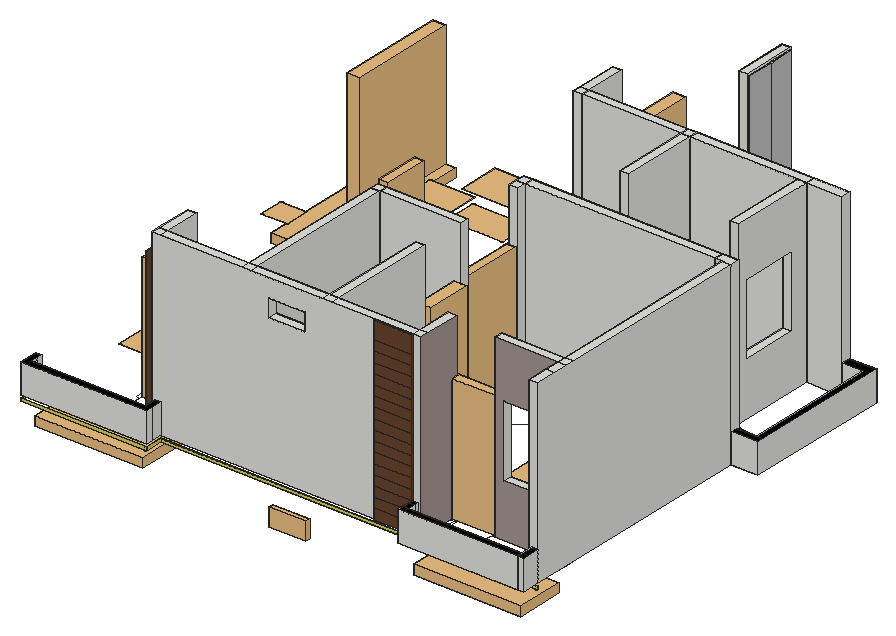
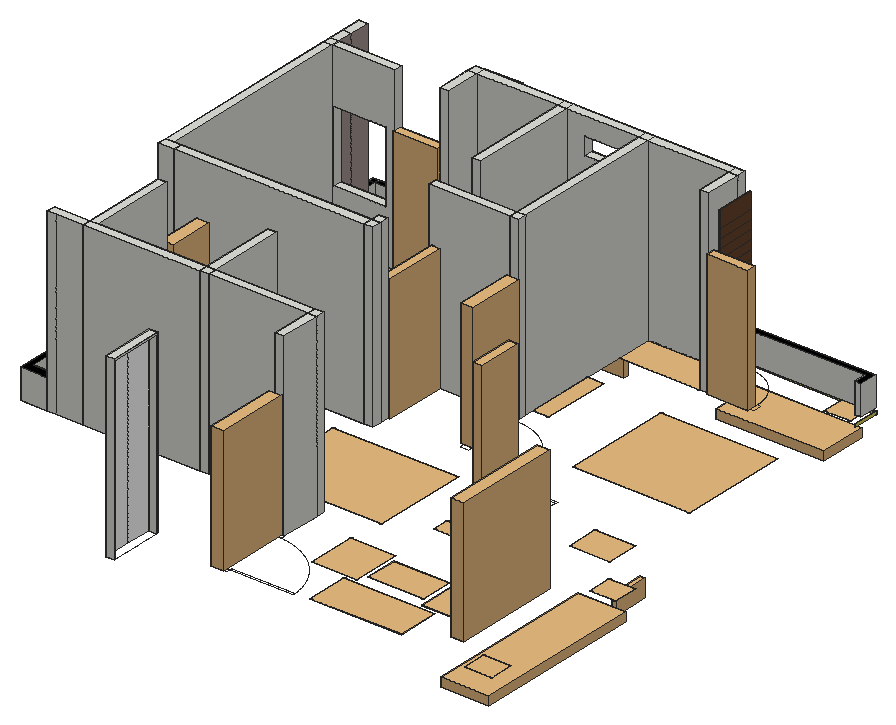
# SketchUp Ruby script. Lengths in inches.
U = 1.inch
M = Sketchup.active_model
def pt(a) = Geom::Point3d.new(a.map { |v| v * U })
def face(e, loops, mat)
  f = e.add_face(loops[0].map { |a| pt(a) })
  loops[1..].each { |l| e.add_face(l.map { |a| pt(a) }).erase! }
  f.material = f.back_material = mat if mat
  f
end
# faces: each face lists its corners as indices into pts; further lists are holes
def faces(e, pts, list, mat = nil) = list.each { |f| face(e, (f[0].is_a?(Array) ? f : [f]).map { |l| l.map { |i| pts[i] } }, mat) }
# xy, xz, yz: faces in a plane at the given z, y or x. An outline is a flat list of corners, or four numbers for a rectangle; further outlines are holes
def ring(l) = l.size == 4 ? [[l[0], l[1]], [l[2], l[1]], [l[2], l[3]], [l[0], l[3]]] : l.each_slice(2).to_a
def flat(e, list, mat, &to3) = list.each { |f| face(e, (f[0].is_a?(Array) ? f : [f]).map { |l| ring(l).map { |u, v| to3.(u, v) } }, mat) }
def xy(e, z, list, mat = nil) = flat(e, list, mat) { |x, y| [x, y, z] }
def xz(e, y, list, mat = nil) = flat(e, list, mat) { |x, z| [x, y, z] }
def yz(e, x, list, mat = nil) = flat(e, list, mat) { |y, z| [x, y, z] }
def lines(e, pts, list) = list.each { |a, b| e.add_line(pt(pts[a]), pt(pts[b])) }
# prism: a flat outline (further loops are holes) pulled along v
def prism(e, loops, v, mat = nil)
  f = face(e, loops, mat); d = Geom::Vector3d.new(v.map { |x| x * U })
  f.pushpull(f.normal.samedirection?(d) ? d.length : -d.length)
end
def box(e, o, s, mat = nil) = prism(e, [[o, [o[0] + s[0], o[1], o[2]], [o[0] + s[0], o[1] + s[1], o[2]], [o[0], o[1] + s[1], o[2]]]], [0, 0, s[2]], mat)
def at(x, y, z, deg = 0) = Geom::Transformation.translation(pt([x, y, z])) * Geom::Transformation.rotation(ORIGIN, Z_AXIS, deg.degrees)
def axes(o, x, y, z) = Geom::Transformation.new([*x, 0, *y, 0, *z, 0, *pt(o).to_a, 1])
def part(name) = M.definitions.add(name)
# library, detail: a bought-in or finely detailed component or shape, given as its bounding box
def library(name, o, s) = part(name).tap { |d| box(d.entities, o, s) }
def detail(e, o, s) = box(e.add_group.entities, o, s)
def put(e, d, t, mat = nil) = e.add_instance(d, t).tap { |i| i.material = mat if mat }
def group(e, t, mat = nil) = e.add_group.tap { |g| g.transformation = t; g.material = mat if mat }.entities
root = M.entities
M.materials.add("0-SS4").color = [255, 255, 255]
M.materials.add("0-SS7").color = [192, 192, 192]
M.materials.add("0-grey 3").color = [204, 204, 204]
M.materials.add("2121 AP  X165 Dhaani-I").color = [217, 210, 92]
M.materials.add("M09_Shadow_Night").color = [0, 0, 0]
M.materials.add("Marble_06_1K").color = [165, 150, 147]
M.materials.add("Wood_Veneer_15_1K").color = [103, 69, 45]
c1 = part("Group\#6")
xy(c1.entities,0,[[0,-8,80,-4],[80,-8,84,-4],[0,-4,4,0],[80,-4,84,4],[0,0,4,4]])
xy(c1.entities,20,[[0,-8,84,-8,84,4,80,4,80,-4,4,-4,4,4,0,4]],"M09_Shadow_Night")
xz(c1.entities,-8,[[0,0,84,20]])
xz(c1.entities,-4,[[4,0,80,20]])
xz(c1.entities,4,[[0,0,4,20],[80,0,84,20]])
yz(c1.entities,0,[[-8,0,4,20]])
yz(c1.entities,4,[[-4,0,0,20],[0,0,4,20]])
yz(c1.entities,80,[[-4,0,4,20]])
yz(c1.entities,84,[[-8,0,-4,20],[-4,0,4,20]])
c2 = part("Group\#8")
xy(c2.entities,0,[[0,-8.88,4,-4.88],[4,-8.88,80,-4.88],[80,-8.88,84,-4.88],[0,-4.88,4,0],[80,-4.88,84,3.12],
  [0,0,4,3.12]])
xy(c2.entities,20,[[0,-8.88,4,-4.88],[4,-8.88,80,-4.88],[80,-8.88,84,-4.88],[0,-4.88,4,0],[80,-4.88,84,3.12],
  [0,0,4,3.12]],"M09_Shadow_Night")
xz(c2.entities,-8.88,[[0,0,80,20],[80,0,84,20]])
xz(c2.entities,-4.88,[[4,0,80,20]])
xz(c2.entities,3.12,[[0,0,4,20],[80,0,84,20]])
yz(c2.entities,0,[[-8.88,0,3.12,20]])
yz(c2.entities,4,[[-4.88,0,0,20],[0,0,3.12,20]])
yz(c2.entities,80,[[-8.88,0,-4.88,20],[-4.88,0,3.12,20]])
yz(c2.entities,84,[[-8.88,0,3.12,20]])
c3 = part("Group\#144")
xy(c3.entities,0,[[0,0,84.5,0.1],[84.5,0,84.6,0.1],[0,0.1,0.5,17.21],[84.5,0.1,84.5,12.09,336.84,12.09,336.84,11.99,84.6,11.99,84.6,0.1]])
xy(c3.entities,2,[[0,0,84.5,0.1],[84.5,0,84.6,0.1],[0,0.1,0.5,17.21],[84.5,0.1,84.6,0.1,84.6,11.99,336.84,11.99,336.84,12.09,84.5,12.09]])
xz(c3.entities,0,[[0,0,84.5,2],[84.5,0,84.6,2]])
xz(c3.entities,0.1,[[0,0,0.5,2],[0.5,0,84.5,2],[84.5,0,84.6,2]])
xz(c3.entities,11.99,[[84.6,0,252.77,2],[252.77,0,336.84,2]])
xz(c3.entities,12.09,[[84.5,0,336.84,2]])
xz(c3.entities,17.21,[[0,0,0.5,2]])
yz(c3.entities,0,[[0,0,0.1,2],[0.1,0,17.21,2]])
yz(c3.entities,0.5,[[0.1,0,17.21,2]])
yz(c3.entities,84.5,[[0,0,0.1,2],[0.1,0,12.09,2]])
yz(c3.entities,84.6,[[0,0,0.1,2],[0.1,0,11.99,2]])
yz(c3.entities,336.84,[[11.99,0,12.09,2]])
c4 = library("TREE-26",[-60.96,-72.91,0],[121.92,134.74,0.01])
c5 = part("Group\#116")
xy(c5.entities,0,[[24,0,24.75,24.75]])
xy(c5.entities,107,[[24,0,24.75,24.75]])
xz(c5.entities,0,[[24,0,24.75,107]])
xz(c5.entities,24.75,[[24,0,24.75,107]])
yz(c5.entities,24,[[0,0,24.75,6],[0,6,24.75,12],[0,12,24.75,18],[0,18,24.75,24],[0,24,24.75,30],
  [0,30,24.75,36],[0,36,24.75,42],[0,42,24.75,48],[0,48,24.75,54],[0,54,24.75,60],
  [0,60,24.75,66],[0,66,24.75,72],[0,72,24.75,78],[0,78,24.75,84],[0,84,24.75,90],
  [0,90,24.75,96],[0,96,24.75,107]],"Wood_Veneer_15_1K")
yz(c5.entities,24.75,[[0,0,24.75,107]])
c6 = library("Group\#46",[0,-0.05,0],[30,2.55,24])
c7 = library("Group\#115",[0,0,0],[72,16,6.2])
c8 = part("tgr")
p = [[-2.37,-3.35,0],[-2.37,-2.82,0],[-2.73,-2.82,0],[-2.73,-2.68,0],[-3.71,-2.68,0],[-3.71,-3.35,0],
  [-2.37,3.35,0],[-2.37,2.82,0],[-2.73,2.82,0],[-2.73,2.68,0],[-3.71,2.68,0],[-3.71,3.35,0],
  [3.71,-2.82,0],[-2.37,-2.46,0],[3.71,-2.46,0],[3.7,-2.46,0],[3.63,-2.07,0],[3.53,-1.68,0],
  [3.41,-1.3,0],[3.27,-0.93,0],[3.1,-0.57,0],[2.91,-0.22,0],[2.7,0.12,0],[2.46,0.4375,0],
  [2.21,0.74,0],[1.93,1.03,0],[1.64,1.3,0],[1.33,1.55,0],[1.01,1.79,0],[0.67,1.99,0],
  [0.32,2.18,0],[-0.04,2.35,0],[-0.41,2.49,0],[-0.8,2.6,0],[-1.18,2.69,0],[-1.58,2.76,0],
  [-1.97,2.8,0]]
lines(c8.entities,p,[[0,1],[1,2],[2,3],[3,4],[4,5],[5,0],[6,7],[7,8],[8,9],[9,10],[10,11],[11,6],
  [1,12],[13,14],[1,13],[12,14],[15,16],[16,17],[17,18],[18,19],[19,20],[20,21],[21,22],[22,23],
  [23,24],[24,25],[25,26],[26,27],[27,28],[28,29],[29,30],[30,31],[31,32],[32,33],[33,34],[34,35],
  [35,36],[36,7]])
c9 = library("Component\#1",[961.32,38.58,0],[54,24,0.01])
c10 = library("Component\#2",[1075.72,38.58,0],[54,24,0.01])
c11 = library("ghgjg",[-265.23,-341.01,0],[530.46,682.02,0.01])
c12 = library("Group\#51",[0,0,0],[6.9375,42,86.5])
c13 = part("GTGTGYHYHYHY")
p = [[-3.29,3.76,0],[3.29,3.76,0],[3.29,-3.76,0],[-3.29,-3.76,0]]
lines(c13.entities,p,[[0,1],[1,2],[2,3],[3,0],[0,2],[1,3]])
c14 = part("G5GTGTGT")
p = [[0.52,4.97,0],[0.52,-4.97,0],[0.36,-4.97,0],[0.36,4.97,0],[-0.08,-4.53,0],[-0.08,4.53,0],
  [0.33,4.97,0],[0.3,4.97,0],[0.28,4.96,0],[0.25,4.96,0],[0.22,4.95,0],[0.2,4.94,0],
  [0.17,4.93,0],[0.15,4.92,0],[0.12,4.9,0],[0.1,4.89,0],[0.08,4.87,0],[0.06,4.85,0],
  [0.04,4.83,0],[0.02,4.8125,0],[0,4.79,0],[-0.01,4.77,0],[-0.03,4.74,0],[-0.04,4.72,0],
  [-0.05,4.69,0],[-0.0625,4.67,0],[-0.07,4.64,0],[-0.08,4.61,0],[-0.08,4.59,0],[-0.08,4.56,0],
  [-0.08,-4.56,0],[-0.08,-4.59,0],[-0.08,-4.61,0],[-0.07,-4.64,0],[-0.0625,-4.67,0],[-0.05,-4.69,0],
  [-0.04,-4.72,0],[-0.03,-4.74,0],[-0.01,-4.77,0],[0,-4.79,0],[0.02,-4.8125,0],[0.04,-4.83,0],
  [0.06,-4.85,0],[0.08,-4.87,0],[0.1,-4.89,0],[0.12,-4.9,0],[0.15,-4.92,0],[0.17,-4.93,0],
  [0.2,-4.94,0],[0.22,-4.95,0],[0.25,-4.96,0],[0.28,-4.96,0],[0.3,-4.97,0],[0.33,-4.97,0],
  [-0.08,-1.38,0],[-0.52,-1.38,0],[-0.08,1.38,0],[-0.52,1.38,0]]
lines(c14.entities,p,[[0,1],[1,2],[2,3],[3,0],[4,5],[3,6],[6,7],[7,8],[8,9],[9,10],[10,11],[11,12],
  [12,13],[13,14],[14,15],[15,16],[16,17],[17,18],[18,19],[19,20],[20,21],[21,22],[22,23],[23,24],
  [24,25],[25,26],[26,27],[27,28],[28,29],[29,5],[4,30],[30,31],[31,32],[32,33],[33,34],[34,35],
  [35,36],[36,37],[37,38],[38,39],[39,40],[40,41],[41,42],[42,43],[43,44],[44,45],[45,46],[46,47],
  [47,48],[48,49],[49,50],[50,51],[51,52],[52,53],[53,2],[54,55],[56,57],[55,57]])
c15 = library("lcd-01",[-577.99,-134.75,0],[1155.98,269.5,0.01])
c16 = library("Group\#49",[0,0,0],[8.31,30,84])
c17 = library("JEEW",[-211.14,-299.86,0],[422.28,599.72,0.01])
c18 = library("double bed",[-999.9375,-1062.5,0],[1999.875,2125,0.01])
c19 = part("EGWF")
p = [[2.59,-3.49,0],[2.59,-3.09,0],[2.85,-3.09,0],[2.85,-2.99,0],[3.58,-2.99,0],[3.58,-3.49,0],
  [2.59,3.49,0],[2.59,3.09,0],[2.85,3.09,0],[2.85,2.99,0],[3.58,2.99,0],[3.58,3.49,0],
  [-3.58,-3.09,0],[2.59,-2.82,0],[-3.58,-2.82,0],[2.2,3.07,0],[1.81,3.04,0],[1.42,2.97,0],
  [1.03,2.89,0],[0.66,2.78,0],[0.29,2.64,0],[-0.07,2.48,0],[-0.42,2.3,0],[-0.76,2.1,0],
  [-1.08,1.875,0],[-1.39,1.63,0],[-1.68,1.37,0],[-1.96,1.09,0],[-2.21,0.79,0],[-2.45,0.48,0],
  [-2.67,0.15,0],[-2.86,-0.1875,0],[-3.04,-0.54,0],[-3.1875,-0.9,0],[-3.32,-1.28,0],[-3.42,-1.66,0],
  [-3.5,-2.04,0],[-3.55,-2.43,0]]
lines(c19.entities,p,[[0,1],[1,2],[2,3],[3,4],[4,5],[5,0],[6,7],[7,8],[8,9],[9,10],[10,11],[11,6],
  [1,12],[13,14],[1,13],[12,14],[7,15],[15,16],[16,17],[17,18],[18,19],[19,20],[20,21],[21,22],
  [22,23],[23,24],[24,25],[25,26],[26,27],[27,28],[28,29],[29,30],[30,31],[31,32],[32,33],[33,34],
  [34,35],[35,36],[36,37],[37,14]])
c20 = library("Group\#50",[0,0,0],[6.9375,42,86.5])
c21 = part("Group\#10")
xy(c21.entities,0,[[-133.3,-6,-127.3,0],[-133.3,0,-127.3,6],[-127.3,0,0,6],[0,0,10.7,6]])
xy(c21.entities,120,[[-133.3,-6,-127.3,0],[-133.3,0,-127.3,6],[-127.3,0,0,6],[0,0,10.7,6]])
xz(c21.entities,-6,[[-133.3,0,-127.3,120]])
xz(c21.entities,0,[[-133.3,0,-127.3,120],[-127.3,0,0,120],[0,0,10.7,120]])
xz(c21.entities,6,[[-133.3,0,-127.3,120],[-127.3,0,0,120],[0,0,10.7,120]])
yz(c21.entities,-133.3,[[-6,0,0,120],[0,0,6,120]])
yz(c21.entities,-127.3,[[-6,0,0,120],[0,0,6,120]])
yz(c21.entities,0,[[0,0,6,120]])
yz(c21.entities,10.7,[[0,0,6,120]])
c22 = library("A$C72E23588",[-1177.7,-903.95,0],[2355.4,1807.9,0.01])
c23 = part("Group\#11")
xy(c23.entities,0,[[0,0,5.15,4],[5.15,0,13.95,4],[13.95,0,18,4],[13.95,4,18,93],[-30,36,-24,93],
  [-108,42,-102,93],[-180.4,93,-174.4,99],[-174.4,93,-108,99],[-108,93,-102,99],[-102,93,-24,99],
  [-24,93,-6,99],[-6,93,0,99],[0,93,13.95,99],[13.95,93,18,99],[-180.4,99,-174.4,126.21]])
xy(c23.entities,20,[[0,0,18,4],[13.95,4,18,4,18,99,0,99,0,93,13.95,93]],"M09_Shadow_Night")
xy(c23.entities,36,[[-30,42,-24,81]])
xy(c23.entities,84,[[-30,42,-24,81]])
xy(c23.entities,120,[[-30,36,-24,93],[-108,42,-102,93],[-180.4,93,-174.4,99],[-174.4,93,-108,99],[-108,93,-102,99],
  [-102,93,-24,99],[-24,93,0,99],[-180.4,99,-174.4,126.21]])
xz(c23.entities,0,[[0,0,18,20]])
xz(c23.entities,4,[[0,0,5.15,20],[5.15,0,13.95,20]])
xz(c23.entities,36,[[-30,0,-24,120]])
xz(c23.entities,42,[[-108,0,-102,120],[-30,36,-24,84]])
xz(c23.entities,81,[[-30,36,-24,84]])
xz(c23.entities,93,[[-180.4,0,-174.4,120],[-174.4,0,-108,120],[-108,0,-102,120],[-102,0,-30,120],[-30,0,-24,120],
  [-24,0,0,120],[0,0,13.95,20]])
xz(c23.entities,99,[[-180.4,0,-174.4,120],[-174.4,0,-108,120],[-108,0,-102,120],[-102,0,-24,120],[-24,0,-6,120],
  [-6,0,0,120],[0,0,18,20]])
xz(c23.entities,126.21,[[-180.4,0,-174.4,120]])
yz(c23.entities,-180.4,[[93,0,99,120],[99,0,126.21,120]])
yz(c23.entities,-174.4,[[93,0,99,120],[99,0,126.21,120]])
yz(c23.entities,-108,[[42,0,93,120],[93,0,99,120]])
yz(c23.entities,-102,[[42,0,93,120],[93,0,99,120]])
yz(c23.entities,-30,[[[36,0,93,120],[42,36,81,84]]])
yz(c23.entities,-24,[[[36,0,93,120],[42,36,81,84]],[93,0,99,120]])
yz(c23.entities,0,[[0,0,4,20],[93,0,99,20],[93,20,99,120]])
yz(c23.entities,13.95,[[4,0,93,20]])
yz(c23.entities,18,[[0,0,99,20]])
c24 = library("porta correr aluminio",[0,0,0],[4.49,110.28,83.35])
c25 = library("BFGFV",[-4.32,-2.51,0],[8.64,5.02,0.01])
c26 = library("VVVV",[-3.39,-3.68,0],[6.78,7.36,0.01])
c27 = part("feeeeeeeeee")
p = [[-2.68,3.51,0],[-2.68,3.16,0],[-2.92,3.16,0],[-2.92,3.07,0],[-3.56,3.07,0],[-3.56,3.51,0],
  [-2.68,-3.51,0],[-2.68,-3.16,0],[-2.92,-3.16,0],[-2.92,-3.07,0],[-3.56,-3.07,0],[-3.56,-3.51,0],
  [3.56,3.16,0],[-2.68,2.93,0],[3.56,2.93,0],[-2.48,-3.13,0],[-2.04,-3.07,0],[-1.61,-2.98,0],
  [-1.1875,-2.86,0],[-0.77,-2.72,0],[-0.36,-2.55,0],[0.03,-2.35,0],[0.41,-2.13,0],[0.78,-1.88,0],
  [1.125,-1.62,0],[1.46,-1.32,0],[1.77,-1.01,0],[2.06,-0.68,0],[2.33,-0.33,0],[2.57,0.03,0],
  [2.79,0.42,0],[2.99,0.81,0],[3.16,1.22,0],[3.3,1.63,0],[3.41,2.06,0],[3.5,2.49,0]]
lines(c27.entities,p,[[0,1],[1,2],[2,3],[3,4],[4,5],[5,0],[6,7],[7,8],[8,9],[9,10],[10,11],[11,6],
  [1,12],[13,14],[1,13],[12,14],[8,15],[15,16],[16,17],[17,18],[18,19],[19,20],[20,21],[21,22],
  [22,23],[23,24],[24,25],[25,26],[26,27],[27,28],[28,29],[29,30],[30,31],[31,32],[32,33],[33,34],
  [34,35],[35,14]])
c28 = library("HYHHYHYHYHYHY",[-2.09,-4.54,0],[4.18,9.08,0.01])
c29 = part("Lift Door")
g1 = group(c29.entities,at(22.98,-1.97,0))
xy(g1,0,[[-11.49,0,22.98,1.97]],"0-SS7")
xy(g1,81.69,[[-11.49,0,22.98,1.97]],"0-SS7")
xz(g1,0,[[-11.49,0,22.98,81.69]],"0-SS7")
xz(g1,1.97,[[-11.49,0,22.98,81.69]],"0-SS4")
yz(g1,-11.49,[[0,0,1.97,81.69]],"0-SS7")
yz(g1,22.98,[[0,0,1.97,81.69]],"0-SS7")
c30 = part("Group\#83")
put(c30.entities,c29,axes([5.4,10.39,0],[0,0.42899,0],[-0.53123,0,0],[0,0,1.07229]),"0-grey 3")
put(c30.entities,c29,axes([5.4,-4.4,0],[0,0.42899,0],[-0.53123,0,0],[0,0,1.07229]),"0-grey 3")
g2 = group(c30.entities,at(0,44.39,0))
p = [[0,-44.39,88.58],[0,-13.75,88.58],[0,-13.75,0],[0,-44.39,0]]
lines(g2,p,[[0,1],[1,2],[3,0],[2,3]])
g3 = group(c30.entities,at(2.42,30.63,0))
prism(g3,[[[2.98,-30.63,0],[2.98,-30.11,0],[2.98,-30.11,87.6],[2.98,-0.53,87.6],[2.98,-0.53,0],[2.98,0,0],[2.98,0,88.58],[2.98,-30.63,88.58]]],[-5.4,0,0])
xy(root,246,[[109.8,55.34,163.8,79.34],[224.2,55.34,278.2,79.1]])
put(root,c1,at(25.8,45.34,246))
put(root,c2,at(278.2,46.22,246))
put(root,c3,at(25.3,37.24,242.13),"2121 AP  X165 Dhaani-I")
put(root,c4,axes([36.72,48.3,246],[0,0.1317,0],[0.1317,0,0],[0,0,0.1317]))
put(root,c4,axes([350.625,48.65,246],[0,0.1317,0],[0.1317,0,0],[0,0,0.1317]))
put(root,c5,axes([278.2,24.59,246],[0,1,0],[-1.02586,0,0],[0,0,1.1215]),"Wood_Veneer_15_1K")
put(root,c6,axes([181.8,50.02,216],[0.81333,0,0],[0,1.27878,0],[0,0,0.5]))
put(root,c7,axes([31.8,41.34,234],[1,0,0],[0,2,0],[0,0,-1]))
put(root,c7,axes([285.28,41.34,233.86],[1,0,0],[0,2,0],[0,0,-1]))
put(root,c5,axes([77.05,47.74,246.5],[1,0,0],[0,1.02586,0],[0,0,1.00467]),"Wood_Veneer_15_1K")
put(root,c8,axes([299.2,62.74,246],[0,-4.47464,0],[4.47464,0,0],[0,0,4.47464]))
put(root,c8,axes([88.8,62.74,246],[0,-4.47464,0],[-4.47464,0,0],[0,0,4.47464]))
put(root,c9,at(-851.52,16.76,246))
put(root,c10,at(-851.52,16.76,246))
put(root,c11,axes([194,68.98,246],[0.04,0,0],[0,-0.04,0],[0,0,0.04]))
put(root,c12,axes([284.2,81,246],[0,-0.85622,0],[0.71429,0,0],[0,0,0.9711]))
put(root,c12,axes([76.2,81,246],[0,-0.85622,0],[0.65714,0,0],[0,0,0.9711]))
put(root,c13,axes([330.2,104.34,246],[0,-2.12603,0],[2.12603,0,0],[0,0,2.12603]))
g4 = group(root,at(103.8,49.34,246))
xy(g4,0,[[0,0,6,6],[6,0,60,6],[60,0,66,6],[66,0,114.4,6],[114.4,0,120.4,6],
  [120.4,0,174.4,6],[174.4,0,180.4,6],[0,6,6,30],[60,6,66,108],[114.4,6,120.4,78],
  [174.4,6,180.4,30],[60,108,66,114],[66,108,120.4,114]])
xy(g4,96,[[78,0,102.4,6]])
xy(g4,108,[[78,0,102.4,6]])
xy(g4,120,[[0,0,6,6],[6,0,60,6],[60,0,66,6],[66,0,114.4,6],[114.4,0,120.4,6],
  [120.4,0,174.4,6],[174.4,0,180.4,6],[0,6,6,30],[60,6,66,108],[114.4,6,120.4,78],
  [174.4,6,180.4,30],[60,108,66,114],[66,108,120.4,114]])
xz(g4,0,[[[0,0,180.4,120],[78,96,102.4,108]]])
xz(g4,6,[[0,0,6,120],[6,0,60,120],[60,0,66,120],[[66,0,114.4,120],[78,96,102.4,108]],[114.4,0,120.4,120],
  [120.4,0,174.4,120]])
xz(g4,30,[[0,0,6,120],[174.4,0,180.4,120]])
xz(g4,78,[[114.4,0,120.4,120]])
xz(g4,108,[[60,0,66,120],[66,0,120.4,120]])
xz(g4,114,[[60,0,66,120],[66,0,120.4,120]])
yz(g4,0,[[0,0,6,120],[6,0,30,120]])
yz(g4,6,[[6,0,30,120]])
yz(g4,60,[[6,0,108,120],[108,0,114,120]])
yz(g4,66,[[6,0,108,120],[108,0,114,120]])
yz(g4,78,[[0,96,6,108]])
yz(g4,102.4,[[0,96,6,108]])
yz(g4,114.4,[[6,0,78,120]])
yz(g4,120.4,[[6,0,78,120],[108,0,114,120]])
yz(g4,174.4,[[6,0,30,120]])
yz(g4,180.4,[[0,0,30,120]],"Marble_06_1K")
put(root,c14,axes([226.1,107.57,246],[3.62,0,0],[0,3.62,0],[0,0,3.62]))
put(root,c15,axes([158.41,128.75,246],[0,-0.04,0],[0.04,0,0],[0,0,0.04]))
g5 = group(root,at(356.2,49.34,246))
xy(g5,0,[[0,0,6,13.86],[0,13.86,6,24],[-42,24,0,30],[0,24,6,30],[0,30,6,162]])
xy(g5,36,[[-36,24,-1,30]])
xy(g5,84,[[-36,24,-1,30]])
xy(g5,120,[[0,0,6,13.86],[0,13.86,6,24],[-42,24,0,30],[0,24,6,30],[0,30,6,162]])
xz(g5,0,[[0,0,6,120]])
xz(g5,24,[[[-42,0,0,120],[-36,36,-1,84]]],"Marble_06_1K")
xz(g5,30,[[[-42,0,0,120],[-36,36,-1,84]]])
xz(g5,162,[[0,0,6,120]])
yz(g5,-42,[[24,0,30,120]])
yz(g5,-36,[[24,36,30,84]])
yz(g5,-1,[[24,36,30,84]])
yz(g5,0,[[24,0,30,120],[30,0,162,120]])
yz(g5,0,[[0,0,13.86,120],[13.86,0,24,120]],"Marble_06_1K")
yz(g5,6,[[0,0,162,120]])
put(root,c8,axes([207.6,142.34,246],[-4.47464,0,0],[0,-4.47464,0],[0,0,4.47464]))
put(root,c16,at(219.92,127.34,246))
put(root,c17,axes([178.84,144.49,246],[-0.04284,0,0],[0,0.04284,0],[0,0,0.04284]))
put(root,c18,axes([316.9375,148.2,246],[0,-0.03695,0],[0.03695,0,0],[0,0,0.03695]))
put(root,c18,axes([71.06,148.29,246],[0,-0.03695,0],[-0.03695,0,0],[0,0,0.03695]))
put(root,c16,axes([163.72,163.34,246],[1,0,0],[0,1.28434,0],[0,0,1]))
put(root,c19,axes([148.2,184.34,246],[6.02515,0,0],[0,-6.02515,0],[0,0,6.02515]))
put(root,c20,axes([216.54,163.34,246],[0.85622,0,0],[0,1,0],[0,0,0.9711]))
put(root,c19,axes([239.8,184.34,246],[-6.02515,0,0],[0,-6.02515,0],[0,0,6.02515]))
put(root,c21,at(351.5,211.34,246))
put(root,c16,axes([336.48,247.16,246],[-1,0,0],[0,-0.994,0],[0,0,1]))
put(root,c8,axes([109.2,232.34,246],[-4.47464,0,0],[0,4.47464,0],[0,0,4.47464]))
put(root,c12,axes([127.46,247.34,246],[-0.85622,0,0],[0,-0.71429,0],[0,0,0.9711]))
put(root,c8,axes([348.8,232.34,246],[4.47464,0,0],[0,4.47464,0],[0,0,4.47464]))
put(root,c11,axes([45.4375,241.34,246],[0,-0.04,0],[-0.04,0,0],[0,0,0.04]))
put(root,c6,axes([26.6,253.34,216],[0,-0.8,0],[1.27878,0,0],[0,0,0.5]))
put(root,c17,axes([106.95,256.29,246],[0,0.04284,0],[0.04284,0,0],[0,0,0.04284]))
put(root,c22,axes([191.83,263.52,246],[0.0356,0,0],[0,-0.0356,0],[0,0,0.0356]))
put(root,c23,at(362.2,211.34,246))
put(root,c4,axes([12.58,274.84,246],[0,0.1317,0],[0.1317,0,0],[0,0,0.1317]))
put(root,c15,axes([102.68,276.73,246],[0.04,0,0],[0,-0.04,0],[0,0,0.04]))
put(root,c7,axes([5.8,385.9,233.5],[0,-1.5912,0],[2,0,0],[0,0,-1]))
put(root,c24,axes([45.93,295.34,246.65],[-1.89519,0,0],[0,0.65291,0],[0,0,1]))
put(root,c25,axes([101.4,333.38,246],[4.3395,0,0],[0,-4.3395,0],[0,0,4.3395]))
put(root,c26,axes([64.42,333.77,246],[4.47564,0,0],[0,-4.47564,0],[0,0,4.47564]))
put(root,c26,axes([138,333.77,246],[-4.47564,0,0],[0,-4.47564,0],[0,0,4.47564]))
put(root,c27,axes([163.46,361.55,246],[-6.83664,0,0],[0,6.83664,0],[0,0,6.83664]))
put(root,c16,axes([183.52,337.55,246],[1,0,0],[0,1.6118,0],[0,0,1]))
put(root,c28,axes([99.08,366.86,246],[0,6.75189,0],[6.75189,0,0],[0,0,6.75189]))
put(root,c4,axes([12.58,379.27,246],[0,0.1317,0],[0.1317,0,0],[0,0,0.1317]))
put(root,c30,axes([236.2,375.58,245.39],[1,0,0],[0,1.17593,0],[0,0,1.36155]))
